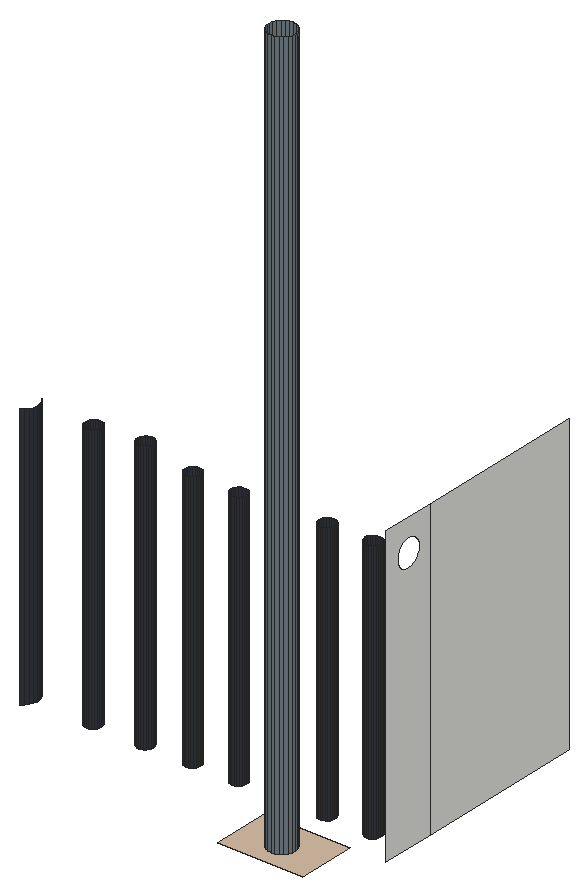
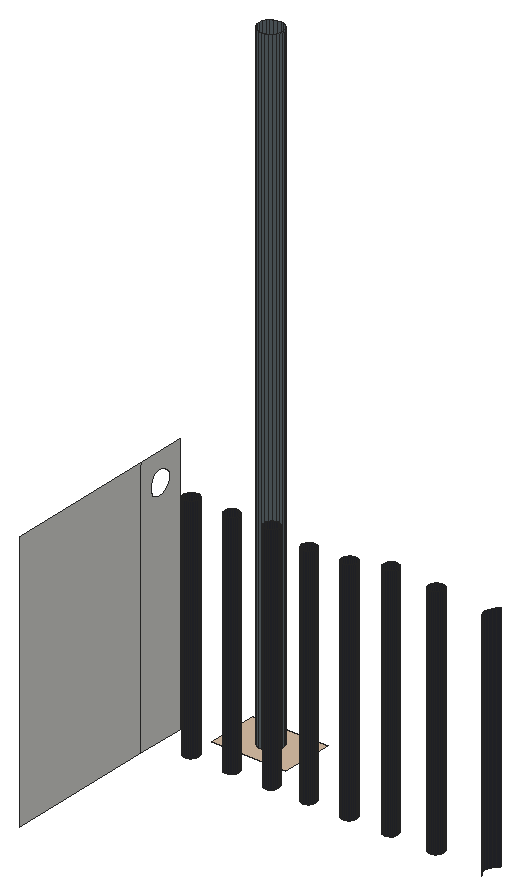
# SketchUp Ruby script. Lengths in inches.
U = 1.inch
M = Sketchup.active_model
def pt(a) = Geom::Point3d.new(a.map { |v| v * U })
def face(e, loops, mat)
  f = e.add_face(loops[0].map { |a| pt(a) })
  loops[1..].each { |l| e.add_face(l.map { |a| pt(a) }).erase! }
  f.material = f.back_material = mat if mat
  f
end
# faces: each face lists its corners as indices into pts; further lists are holes
def faces(e, pts, list, mat = nil) = list.each { |f| face(e, (f[0].is_a?(Array) ? f : [f]).map { |l| l.map { |i| pts[i] } }, mat) }
# xy, xz, yz: faces in a plane at the given z, y or x. An outline is a flat list of corners, or four numbers for a rectangle; further outlines are holes
def ring(l) = l.size == 4 ? [[l[0], l[1]], [l[2], l[1]], [l[2], l[3]], [l[0], l[3]]] : l.each_slice(2).to_a
def flat(e, list, mat, &to3) = list.each { |f| face(e, (f[0].is_a?(Array) ? f : [f]).map { |l| ring(l).map { |u, v| to3.(u, v) } }, mat) }
def xy(e, z, list, mat = nil) = flat(e, list, mat) { |x, y| [x, y, z] }
def xz(e, y, list, mat = nil) = flat(e, list, mat) { |x, z| [x, y, z] }
def yz(e, x, list, mat = nil) = flat(e, list, mat) { |y, z| [x, y, z] }
def lines(e, pts, list) = list.each { |a, b| e.add_line(pt(pts[a]), pt(pts[b])) }
# prism: a flat outline (further loops are holes) pulled along v
def prism(e, loops, v, mat = nil)
  f = face(e, loops, mat); d = Geom::Vector3d.new(v.map { |x| x * U })
  f.pushpull(f.normal.samedirection?(d) ? d.length : -d.length)
end
def box(e, o, s, mat = nil) = prism(e, [[o, [o[0] + s[0], o[1], o[2]], [o[0] + s[0], o[1] + s[1], o[2]], [o[0], o[1] + s[1], o[2]]]], [0, 0, s[2]], mat)
def at(x, y, z, deg = 0) = Geom::Transformation.translation(pt([x, y, z])) * Geom::Transformation.rotation(ORIGIN, Z_AXIS, deg.degrees)
def axes(o, x, y, z) = Geom::Transformation.new([*x, 0, *y, 0, *z, 0, *pt(o).to_a, 1])
def part(name) = M.definitions.add(name)
# library, detail: a bought-in or finely detailed component or shape, given as its bounding box
def library(name, o, s) = part(name).tap { |d| box(d.entities, o, s) }
def detail(e, o, s) = box(e.add_group.entities, o, s)
def put(e, d, t, mat = nil) = e.add_instance(d, t).tap { |i| i.material = mat if mat }
def group(e, t, mat = nil) = e.add_group.tap { |g| g.transformation = t; g.material = mat if mat }.entities
root = M.entities
M.materials.add("[Formica Laminate Dark]").color = [50, 53, 60]
M.materials.add("[Formica Laminate Light]").color = [213, 189, 164]
M.materials.add("[Formica Speckled Grey]").color = [112, 125, 132]
xy(root,479.47,[[368.82,84.97,368.45,85.02,368.11,85.17,367.81,85.4,367.58,85.69,367.4375,86.04,367.39,86.41,367.4375,86.78,367.58,87.13,367.81,87.43,368.11,87.66,368.45,87.8,368.82,87.85,369.2,87.8,369.54,87.66,369.84,87.43,370.07,87.13,370.21,86.78,370.26,86.41,370.21,86.04,370.07,85.69,369.84,85.4,369.54,85.17,369.2,85.02],[343.53,91.9,343.3,91.93,343.09,92.02,342.91,92.16,342.77,92.34,342.68,92.55,342.65,92.78,342.68,93.01,342.77,93.22,342.91,93.4,343.09,93.54,343.3,93.625,343.53,93.65,343.75,93.625,343.97,93.54,344.15,93.4,344.29,93.22,344.375,93.01,344.4,92.78,344.375,92.55,344.29,92.34,344.15,92.16,343.97,92.02,343.75,91.93],[349.09,91.9,348.86,91.93,348.65,92.02,348.47,92.16,348.33,92.34,348.25,92.55,348.22,92.78,348.25,93.01,348.33,93.22,348.47,93.4,348.65,93.54,348.86,93.625,349.09,93.65,349.32,93.625,349.53,93.54,349.71,93.4,349.85,93.22,349.9375,93.01,349.97,92.78,349.9375,92.55,349.85,92.34,349.71,92.16,349.53,92.02,349.32,91.93],[354.15,91.9,353.93,91.93,353.72,92.02,353.53,92.16,353.4,92.34,353.31,92.55,353.28,92.78,353.31,93.01,353.4,93.22,353.53,93.4,353.72,93.54,353.93,93.625,354.15,93.65,354.38,93.625,354.59,93.54,354.77,93.4,354.91,93.22,355,93.01,355.03,92.78,355,92.55,354.91,92.34,354.77,92.16,354.59,92.02,354.38,91.93],[359.09,91.9,358.86,91.93,358.65,92.02,358.47,92.16,358.33,92.34,358.25,92.55,358.22,92.78,358.25,93.01,358.33,93.22,358.47,93.4,358.65,93.54,358.86,93.625,359.09,93.65,359.32,93.625,359.53,93.54,359.71,93.4,359.85,93.22,359.9375,93.01,359.97,92.78,359.9375,92.55,359.85,92.34,359.71,92.16,359.53,92.02,359.32,91.93],
  [363.65,91.9,363.43,91.93,363.22,92.02,363.03,92.16,362.9,92.34,362.81,92.55,362.78,92.78,362.81,93.01,362.9,93.22,363.03,93.4,363.22,93.54,363.43,93.625,363.65,93.65,363.88,93.625,364.09,93.54,364.27,93.4,364.41,93.22,364.5,93.01,364.53,92.78,364.5,92.55,364.41,92.34,364.27,92.16,364.09,92.02,363.88,91.93],[368.53,91.9,368.3,91.93,368.09,92.02,367.91,92.16,367.77,92.34,367.68,92.55,367.65,92.78,367.68,93.01,367.77,93.22,367.91,93.4,368.09,93.54,368.3,93.625,368.53,93.65,368.75,93.625,368.97,93.54,369.15,93.4,369.29,93.22,369.375,93.01,369.4,92.78,369.375,92.55,369.29,92.34,369.15,92.16,368.97,92.02,368.75,91.93],[373.47,91.9,373.24,91.93,373.03,92.02,372.85,92.16,372.71,92.34,372.62,92.55,372.59,92.78,372.62,93.01,372.71,93.22,372.85,93.4,373.03,93.54,373.24,93.625,373.47,93.65,373.69,93.625,373.9,93.54,374.08,93.4,374.22,93.22,374.3125,93.01,374.34,92.78,374.3125,92.55,374.22,92.34,374.08,92.16,373.9,92.02,373.69,91.93]])
xy(root,479.47,[[[364.3,83.42,373.43,89.73],[368.82,84.97,368.45,85.02,368.11,85.17,367.81,85.4,367.58,85.69,367.4375,86.04,367.39,86.41,367.4375,86.78,367.58,87.13,367.81,87.43,368.11,87.66,368.45,87.8,368.82,87.85,369.2,87.8,369.54,87.66,369.84,87.43,370.07,87.13,370.21,86.78,370.26,86.41,370.21,86.04,370.07,85.69,369.84,85.4,369.54,85.17,369.2,85.02]]],"[Formica Laminate Light]")
yz(root,377.32,[[[89.73,479.47,95.64,511.22],[92.71,506.31,93.09,506.36,93.46,506.51,93.77,506.74,94.01,507.06,94.16,507.42,94.21,507.81,94.16,508.19,94.01,508.56,93.77,508.87,93.46,509.1,93.09,509.25,92.71,509.31,92.32,509.25,91.96,509.1,91.65,508.87,91.41,508.56,91.26,508.19,91.21,507.81,91.26,507.42,91.41,507.06,91.65,506.74,91.96,506.51,92.32,506.36]],[95.64,479.47,114.1,511.22]])
p = [[368.11,85.17,479.47],[368.45,85.02,479.47],[368.45,85.02,557.86],[368.11,85.17,557.86],[368.82,84.97,479.47],[368.82,84.97,557.86],
  [369.2,85.02,479.47],[369.2,85.02,557.86],[369.54,85.17,479.47],[369.54,85.17,557.86],[367.81,85.4,479.47],[367.81,85.4,557.86],
  [369.84,85.4,479.47],[369.84,85.4,557.86],[367.58,85.69,479.47],[367.58,85.69,557.86],[370.07,85.69,479.47],[370.07,85.69,557.86],
  [367.4375,86.04,479.47],[367.4375,86.04,557.86],[370.21,86.04,479.47],[370.21,86.04,557.86],[367.39,86.41,479.47],[367.39,86.41,557.86],
  [370.26,86.41,479.47],[370.26,86.41,557.86],[367.4375,86.78,479.47],[367.4375,86.78,557.86],[370.21,86.78,479.47],[370.21,86.78,557.86],
  [367.58,87.13,479.47],[367.58,87.13,557.86],[370.07,87.13,479.47],[370.07,87.13,557.86],[367.81,87.43,479.47],[367.81,87.43,557.86],
  [369.84,87.43,479.47],[369.84,87.43,557.86],[368.11,87.66,479.47],[368.11,87.66,557.86],[369.54,87.66,479.47],[369.54,87.66,557.86],
  [368.45,87.8,479.47],[368.45,87.8,557.86],[369.2,87.8,479.47],[369.2,87.8,557.86],[368.82,87.85,479.47],[368.82,87.85,557.86],
  [336.68,91.53,479.47],[337,91.78,479.47],[337,91.78,507.81],[336.68,91.53,507.81],[337.25,92.1,479.47],[337.25,92.1,507.81],
  [343.09,92.02,479.47],[343.3,91.93,479.47],[343.3,91.93,508.19],[343.09,92.02,508.19],[343.53,91.9,479.47],[343.53,91.9,508.19],
  [343.75,91.93,479.47],[343.75,91.93,508.19],[343.97,92.02,479.47],[343.97,92.02,508.19],[348.65,92.02,479.47],[348.86,91.93,479.47],
  [348.86,91.93,508.56],[348.65,92.02,508.56],[349.09,91.9,479.47],[349.09,91.9,508.56],[349.32,91.93,479.47],[349.32,91.93,508.56],
  [349.53,92.02,479.47],[349.53,92.02,508.56],[353.72,92.02,479.47],[353.93,91.93,479.47],[353.93,91.93,507.41],[353.72,92.02,507.41],
  [354.15,91.9,479.47],[354.15,91.9,507.41],[354.38,91.93,479.47],[354.38,91.93,507.41],[354.59,92.02,479.47],[354.59,92.02,507.41],
  [358.65,92.02,479.47],[358.86,91.93,479.47],[358.86,91.93,507.16],[358.65,92.02,507.16],[359.09,91.9,479.47],[359.09,91.9,507.16],
  [359.32,91.93,479.47],[359.32,91.93,507.16],[359.53,92.02,479.47],[359.53,92.02,507.16],[363.22,92.02,479.47],[363.43,91.93,479.47],
  [363.43,91.93,507.91],[363.22,92.02,507.91],[363.65,91.9,479.47],[363.65,91.9,507.91],[363.88,91.93,479.47],[363.88,91.93,507.91],
  [364.09,92.02,479.47],[364.09,92.02,507.91],[368.09,92.02,479.47],[368.3,91.93,479.47],[368.3,91.93,507.54],[368.09,92.02,507.54],
  [368.53,91.9,479.47],[368.53,91.9,507.54],[368.75,91.93,479.47],[368.75,91.93,507.54],[368.97,92.02,479.47],[368.97,92.02,507.54],
  [373.03,92.02,479.47],[373.24,91.93,479.47],[373.24,91.93,507.6],[373.03,92.02,507.6],[373.47,91.9,479.47],[373.47,91.9,507.6],
  [373.69,91.93,479.47],[373.69,91.93,507.6],[373.9,92.02,479.47],[373.9,92.02,507.6],[342.91,92.16,479.47],[342.91,92.16,508.19],
  [344.15,92.16,479.47],[344.15,92.16,508.19],[348.47,92.16,479.47],[348.47,92.16,508.56],[349.71,92.16,479.47],[349.71,92.16,508.56],
  [353.53,92.16,479.47],[353.53,92.16,507.41],[354.77,92.16,479.47],[354.77,92.16,507.41],[358.47,92.16,479.47],[358.47,92.16,507.16],
  [359.71,92.16,479.47],[359.71,92.16,507.16],[363.03,92.16,479.47],[363.03,92.16,507.91],[364.27,92.16,479.47],[364.27,92.16,507.91],
  [367.91,92.16,479.47],[367.91,92.16,507.54],[369.15,92.16,479.47],[369.15,92.16,507.54],[372.85,92.16,479.47],[372.85,92.16,507.6],
  [374.08,92.16,479.47],[374.08,92.16,507.6],[337.41,92.48,479.47],[337.41,92.48,507.81],[342.77,92.34,479.47],[342.77,92.34,508.19],
  [344.29,92.34,479.47],[344.29,92.34,508.19],[348.33,92.34,479.47],[348.33,92.34,508.56],[349.85,92.34,479.47],[349.85,92.34,508.56],
  [353.4,92.34,479.47],[353.4,92.34,507.41],[354.91,92.34,479.47],[354.91,92.34,507.41],[358.33,92.34,479.47],[358.33,92.34,507.16],
  [359.85,92.34,479.47],[359.85,92.34,507.16],[362.9,92.34,479.47],[362.9,92.34,507.91],[364.41,92.34,479.47],[364.41,92.34,507.91],
  [367.77,92.34,479.47],[367.77,92.34,507.54],[369.29,92.34,479.47],[369.29,92.34,507.54],[372.71,92.34,479.47],[372.71,92.34,507.6],
  [374.22,92.34,479.47],[374.22,92.34,507.6],[342.68,92.55,479.47],[342.68,92.55,508.19],[344.375,92.55,479.47],[344.375,92.55,508.19],
  [348.25,92.55,479.47],[348.25,92.55,508.56],[349.9375,92.55,479.47],[349.9375,92.55,508.56],[353.31,92.55,479.47],[353.31,92.55,507.41],
  [355,92.55,479.47],[355,92.55,507.41],[358.25,92.55,479.47],[358.25,92.55,507.16],[359.9375,92.55,479.47],[359.9375,92.55,507.16],
  [362.81,92.55,479.47],[362.81,92.55,507.91],[364.5,92.55,479.47],[364.5,92.55,507.91],[367.68,92.55,479.47],[367.68,92.55,507.54],
  [369.375,92.55,479.47],[369.375,92.55,507.54],[372.62,92.55,479.47],[372.62,92.55,507.6],[374.3125,92.55,479.47],[374.3125,92.55,507.6],
  [337.46,92.88,479.47],[337.46,92.88,507.81],[342.65,92.78,479.47],[342.65,92.78,508.19],[344.4,92.78,479.47],[344.4,92.78,508.19],
  [348.22,92.78,479.47],[348.22,92.78,508.56],[349.97,92.78,479.47],[349.97,92.78,508.56],[353.28,92.78,479.47],[353.28,92.78,507.41],
  [355.03,92.78,479.47],[355.03,92.78,507.41],[358.22,92.78,479.47],[358.22,92.78,507.16],[359.97,92.78,479.47],[359.97,92.78,507.16],
  [362.78,92.78,479.47],[362.78,92.78,507.91],[364.53,92.78,479.47],[364.53,92.78,507.91],[367.65,92.78,479.47],[367.65,92.78,507.54],
  [369.4,92.78,479.47],[369.4,92.78,507.54],[372.59,92.78,479.47],[372.59,92.78,507.6],[374.34,92.78,479.47],[374.34,92.78,507.6],
  [342.68,93.01,479.47],[342.68,93.01,508.19],[344.375,93.01,479.47],[344.375,93.01,508.19],[348.25,93.01,479.47],[348.25,93.01,508.56],
  [349.9375,93.01,479.47],[349.9375,93.01,508.56],[353.31,93.01,479.47],[353.31,93.01,507.41],[355,93.01,479.47],[355,93.01,507.41],
  [358.25,93.01,479.47],[358.25,93.01,507.16],[359.9375,93.01,479.47],[359.9375,93.01,507.16],[362.81,93.01,479.47],[362.81,93.01,507.91],
  [364.5,93.01,479.47],[364.5,93.01,507.91],[367.68,93.01,479.47],[367.68,93.01,507.54],[369.375,93.01,479.47],[369.375,93.01,507.54],
  [372.62,93.01,479.47],[372.62,93.01,507.6],[374.3125,93.01,479.47],[374.3125,93.01,507.6],[337.41,93.28,479.47],[337.41,93.28,507.81],
  [342.77,93.22,479.47],[342.77,93.22,508.19],[344.29,93.22,479.47],[344.29,93.22,508.19],[348.33,93.22,479.47],[348.33,93.22,508.56],
  [349.85,93.22,479.47],[349.85,93.22,508.56],[353.4,93.22,479.47],[353.4,93.22,507.41],[354.91,93.22,479.47],[354.91,93.22,507.41],
  [358.33,93.22,479.47],[358.33,93.22,507.16],[359.85,93.22,479.47],[359.85,93.22,507.16],[362.9,93.22,479.47],[362.9,93.22,507.91],
  [364.41,93.22,479.47],[364.41,93.22,507.91],[367.77,93.22,479.47],[367.77,93.22,507.54],[369.29,93.22,479.47],[369.29,93.22,507.54],
  [372.71,93.22,479.47],[372.71,93.22,507.6],[374.22,93.22,479.47],[374.22,93.22,507.6],[342.91,93.4,479.47],[342.91,93.4,508.19],
  [344.15,93.4,479.47],[344.15,93.4,508.19],[348.47,93.4,479.47],[348.47,93.4,508.56],[349.71,93.4,479.47],[349.71,93.4,508.56],
  [353.53,93.4,479.47],[353.53,93.4,507.41],[354.77,93.4,479.47],[354.77,93.4,507.41],[358.47,93.4,479.47],[358.47,93.4,507.16],
  [359.71,93.4,479.47],[359.71,93.4,507.16],[363.03,93.4,479.47],[363.03,93.4,507.91],[364.27,93.4,479.47],[364.27,93.4,507.91],
  [367.91,93.4,479.47],[367.91,93.4,507.54],[369.15,93.4,479.47],[369.15,93.4,507.54],[372.85,93.4,479.47],[372.85,93.4,507.6],
  [374.08,93.4,479.47],[374.08,93.4,507.6],[337.25,93.66,479.47],[337.25,93.66,507.81],[343.09,93.54,479.47],[343.09,93.54,508.19],
  [343.97,93.54,479.47],[343.97,93.54,508.19],[348.65,93.54,479.47],[348.65,93.54,508.56],[349.53,93.54,479.47],[349.53,93.54,508.56],
  [353.72,93.54,479.47],[353.72,93.54,507.41],[354.59,93.54,479.47],[354.59,93.54,507.41],[358.65,93.54,479.47],[358.65,93.54,507.16],
  [359.53,93.54,479.47],[359.53,93.54,507.16],[363.22,93.54,479.47],[363.22,93.54,507.91],[364.09,93.54,479.47],[364.09,93.54,507.91],
  [368.09,93.54,479.47],[368.09,93.54,507.54],[368.97,93.54,479.47],[368.97,93.54,507.54],[373.03,93.54,479.47],[373.03,93.54,507.6],
  [373.9,93.54,479.47],[373.9,93.54,507.6],[343.3,93.625,479.47],[343.3,93.625,508.19],[343.75,93.625,479.47],[343.75,93.625,508.19],
  [348.86,93.625,479.47],[348.86,93.625,508.56],[349.32,93.625,479.47],[349.32,93.625,508.56],[353.93,93.625,479.47],[353.93,93.625,507.41],
  [354.38,93.625,479.47],[354.38,93.625,507.41],[358.86,93.625,479.47],[358.86,93.625,507.16],[359.32,93.625,479.47],[359.32,93.625,507.16],
  [363.43,93.625,479.47],[363.43,93.625,507.91],[363.88,93.625,479.47],[363.88,93.625,507.91],[368.3,93.625,479.47],[368.3,93.625,507.54],
  [368.75,93.625,479.47],[368.75,93.625,507.54],[373.24,93.625,479.47],[373.24,93.625,507.6],[373.69,93.625,479.47],[373.69,93.625,507.6],
  [343.53,93.65,479.47],[343.53,93.65,508.19],[349.09,93.65,479.47],[349.09,93.65,508.56],[354.15,93.65,479.47],[354.15,93.65,507.41],
  [359.09,93.65,479.47],[359.09,93.65,507.16],[363.65,93.65,479.47],[363.65,93.65,507.91],[368.53,93.65,479.47],[368.53,93.65,507.54],
  [373.47,93.65,479.47],[373.47,93.65,507.6],[337,93.99,479.47],[337,93.99,507.81]]
faces(root,p,[[0,1,2,3],[1,4,5,2],[4,6,7,5],[6,8,9,7],[10,0,3,11],[8,12,13,9],[14,10,11,15],[12,16,17,13],
  [18,14,15,19],[16,20,21,17],[22,18,19,23],[20,24,25,21],[26,22,23,27],[24,28,29,25],[30,26,27,31],[28,32,33,29],
  [34,30,31,35],[32,36,37,33],[38,34,35,39],[36,40,41,37],[42,38,39,43],[40,44,45,41],[46,42,43,47],[44,46,47,45]],"[Formica Speckled Grey]")
faces(root,p,[[48,49,50,51],[49,52,53,50],[54,55,56,57],[55,58,59,56],[58,60,61,59],[60,62,63,61],[64,65,66,67],[65,68,69,66],
  [68,70,71,69],[70,72,73,71],[74,75,76,77],[75,78,79,76],[78,80,81,79],[80,82,83,81],[84,85,86,87],[85,88,89,86],
  [88,90,91,89],[90,92,93,91],[94,95,96,97],[95,98,99,96],[98,100,101,99],[100,102,103,101],[104,105,106,107],[105,108,109,106],
  [108,110,111,109],[110,112,113,111],[114,115,116,117],[115,118,119,116],[118,120,121,119],[120,122,123,121],[124,54,57,125],[62,126,127,63],
  [128,64,67,129],[72,130,131,73],[132,74,77,133],[82,134,135,83],[136,84,87,137],[92,138,139,93],[140,94,97,141],[102,142,143,103],
  [144,104,107,145],[112,146,147,113],[148,114,117,149],[122,150,151,123],[52,152,153,53],[154,124,125,155],[126,156,157,127],[158,128,129,159],
  [130,160,161,131],[162,132,133,163],[134,164,165,135],[166,136,137,167],[138,168,169,139],[170,140,141,171],[142,172,173,143],[174,144,145,175],
  [146,176,177,147],[178,148,149,179],[150,180,181,151],[182,154,155,183],[156,184,185,157],[186,158,159,187],[160,188,189,161],[190,162,163,191],
  [164,192,193,165],[194,166,167,195],[168,196,197,169],[198,170,171,199],[172,200,201,173],[202,174,175,203],[176,204,205,177],[206,178,179,207],
  [180,208,209,181],[152,210,211,153],[212,182,183,213],[184,214,215,185],[216,186,187,217],[188,218,219,189],[220,190,191,221],[192,222,223,193],
  [224,194,195,225],[196,226,227,197],[228,198,199,229],[200,230,231,201],[232,202,203,233],[204,234,235,205],[236,206,207,237],[208,238,239,209],
  [240,212,213,241],[214,242,243,215],[244,216,217,245],[218,246,247,219],[248,220,221,249],[222,250,251,223],[252,224,225,253],[226,254,255,227],
  [256,228,229,257],[230,258,259,231],[260,232,233,261],[234,262,263,235],[264,236,237,265],[238,266,267,239],[210,268,269,211],[270,240,241,271],
  [242,272,273,243],[274,244,245,275],[246,276,277,247],[278,248,249,279],[250,280,281,251],[282,252,253,283],[254,284,285,255],[286,256,257,287],
  [258,288,289,259],[290,260,261,291],[262,292,293,263],[294,264,265,295],[266,296,297,267],[298,270,271,299],[272,300,301,273],[302,274,275,303],
  [276,304,305,277],[306,278,279,307],[280,308,309,281],[310,282,283,311],[284,312,313,285],[314,286,287,315],[288,316,317,289],[318,290,291,319],
  [292,320,321,293],[322,294,295,323],[296,324,325,297],[268,326,327,269],[328,298,299,329],[300,330,331,301],[332,302,303,333],[304,334,335,305],
  [336,306,307,337],[308,338,339,309],[340,310,311,341],[312,342,343,313],[344,314,315,345],[316,346,347,317],[348,318,319,349],[320,350,351,321],
  [352,322,323,353],[324,354,355,325],[356,328,329,357],[330,358,359,331],[360,332,333,361],[334,362,363,335],[364,336,337,365],[338,366,367,339],
  [368,340,341,369],[342,370,371,343],[372,344,345,373],[346,374,375,347],[376,348,349,377],[350,378,379,351],[380,352,353,381],[354,382,383,355],
  [384,356,357,385],[358,384,385,359],[386,360,361,387],[362,386,387,363],[388,364,365,389],[366,388,389,367],[390,368,369,391],[370,390,391,371],
  [392,372,373,393],[374,392,393,375],[394,376,377,395],[378,394,395,379],[396,380,381,397],[382,396,397,383],[326,398,399,327]],"[Formica Laminate Dark]")
